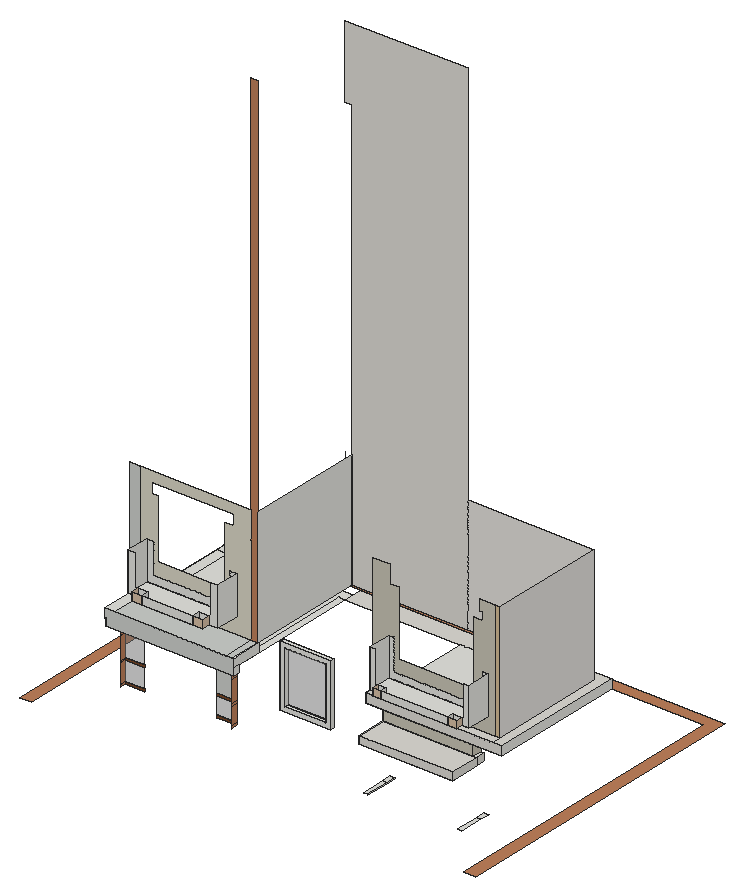
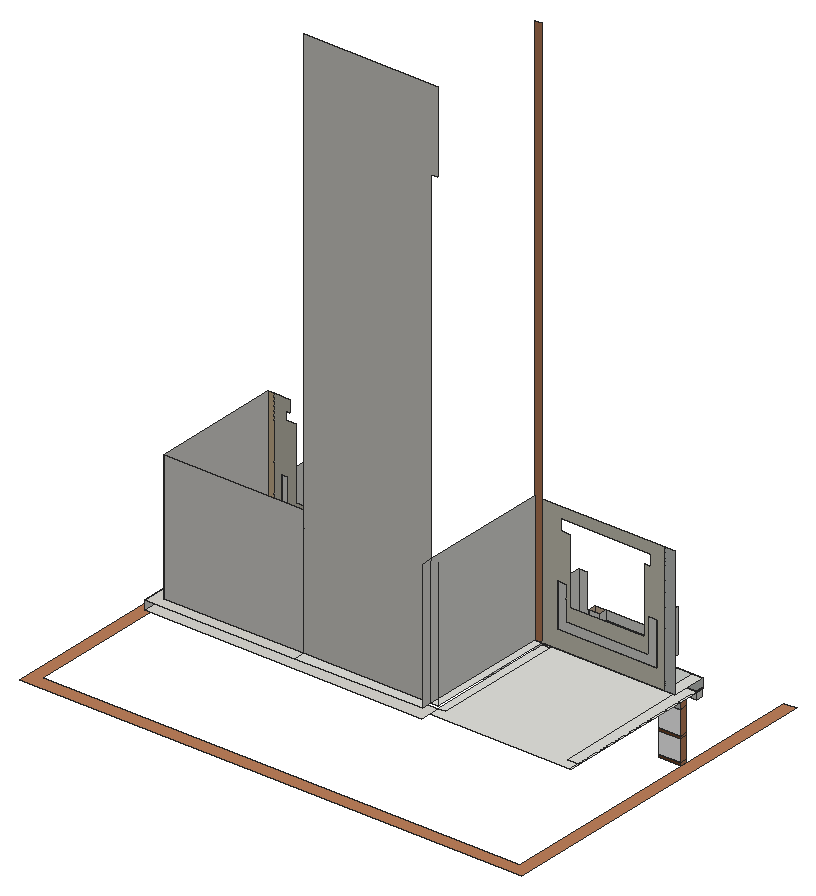
# SketchUp Ruby script. Lengths in inches.
U = 1.inch
M = Sketchup.active_model
def pt(a) = Geom::Point3d.new(a.map { |v| v * U })
def face(e, loops, mat)
  f = e.add_face(loops[0].map { |a| pt(a) })
  loops[1..].each { |l| e.add_face(l.map { |a| pt(a) }).erase! }
  f.material = f.back_material = mat if mat
  f
end
# faces: each face lists its corners as indices into pts; further lists are holes
def faces(e, pts, list, mat = nil) = list.each { |f| face(e, (f[0].is_a?(Array) ? f : [f]).map { |l| l.map { |i| pts[i] } }, mat) }
# xy, xz, yz: faces in a plane at the given z, y or x. An outline is a flat list of corners, or four numbers for a rectangle; further outlines are holes
def ring(l) = l.size == 4 ? [[l[0], l[1]], [l[2], l[1]], [l[2], l[3]], [l[0], l[3]]] : l.each_slice(2).to_a
def flat(e, list, mat, &to3) = list.each { |f| face(e, (f[0].is_a?(Array) ? f : [f]).map { |l| ring(l).map { |u, v| to3.(u, v) } }, mat) }
def xy(e, z, list, mat = nil) = flat(e, list, mat) { |x, y| [x, y, z] }
def xz(e, y, list, mat = nil) = flat(e, list, mat) { |x, z| [x, y, z] }
def yz(e, x, list, mat = nil) = flat(e, list, mat) { |y, z| [x, y, z] }
def lines(e, pts, list) = list.each { |a, b| e.add_line(pt(pts[a]), pt(pts[b])) }
# prism: a flat outline (further loops are holes) pulled along v
def prism(e, loops, v, mat = nil)
  f = face(e, loops, mat); d = Geom::Vector3d.new(v.map { |x| x * U })
  f.pushpull(f.normal.samedirection?(d) ? d.length : -d.length)
end
def box(e, o, s, mat = nil) = prism(e, [[o, [o[0] + s[0], o[1], o[2]], [o[0] + s[0], o[1] + s[1], o[2]], [o[0], o[1] + s[1], o[2]]]], [0, 0, s[2]], mat)
def at(x, y, z, deg = 0) = Geom::Transformation.translation(pt([x, y, z])) * Geom::Transformation.rotation(ORIGIN, Z_AXIS, deg.degrees)
def axes(o, x, y, z) = Geom::Transformation.new([*x, 0, *y, 0, *z, 0, *pt(o).to_a, 1])
def part(name) = M.definitions.add(name)
# library, detail: a bought-in or finely detailed component or shape, given as its bounding box
def library(name, o, s) = part(name).tap { |d| box(d.entities, o, s) }
def detail(e, o, s) = box(e.add_group.entities, o, s)
def put(e, d, t, mat = nil) = e.add_instance(d, t).tap { |i| i.material = mat if mat }
def group(e, t, mat = nil) = e.add_group.tap { |g| g.transformation = t; g.material = mat if mat }.entities
root = M.entities
M.materials.add("[Basic Tile]").color = [203, 206, 202]
M.materials.add("[Formica Beige]").color = [211, 187, 149]
M.materials.add("[Formica Graystone]").color = [198, 194, 180]
M.materials.add("[Formica Graystone]1").color = [216, 212, 196]
M.materials.add("[Formica Laminate Light]").color = [213, 189, 164]
M.materials.add("[Terrazzo Tile Accent]").color = [224, 221, 217]
M.materials.add("[Terrazzo Tile Light]").color = [219, 217, 210]
M.materials.add("[Translucent Glass Gray]").color = [128, 128, 128]
M.materials["[Translucent Glass Gray]"].alpha = 0.5
M.materials.add("[Wood Veneer 01]").color = [120, 70, 37]
M.materials.add("[Wood Veneer 02]").color = [190, 128, 91]
xy(root,63.125,[[288.3125,80.01,293.16,104.39],[384.76,80.01,389.375,104.39],[288.3125,104.39,293.16,114.1],[384.76,104.39,389.375,114.1]])
xy(root,84,[[0,0,11.79,0,11.79,307.53,455.72,307.53,455.72,0,467.51,0,467.51,319.32,0,319.32]],"[Wood Veneer 02]")
xy(root,87.4375,[[179.41,109.54,230.79,114.1]])
xy(root,91.91,[[183.89,109.54,226.3125,114.1]])
xy(root,110.81,[[375.8125,104.39,384.875,114.1]])
xy(root,110.81,[[[289.1875,73.57,384.875,104.39],[377.92,74.4375,378.51,74.59,379.03,74.88,379.47,75.3,379.77,75.82,379.9375,76.4,379.94,77.01,379.8,77.59,379.5,78.12,379.08,78.55,378.56,78.86,377.98,79.02,377.375,79.03,376.79,78.88,376.26,78.58,375.83,78.16,375.52,77.64,375.36,77.0625,375.35,76.46,375.5,75.875,375.8,75.35,376.22,74.92,376.74,74.61,377.32,74.44],[300.49,74.4375,301.07,74.59,301.6,74.88,302.03,75.3,302.34,75.82,302.5,76.4,302.51,77.01,302.36,77.59,302.0625,78.12,301.64,78.55,301.12,78.86,300.54,79.02,299.9375,79.03,299.35,78.88,298.82,78.58,298.39,78.16,298.09,77.64,297.92,77.0625,297.91,76.46,298.0625,75.875,298.36,75.35,298.78,74.92,299.3,74.61,299.88,74.44]],[289.1875,104.39,298,114.1]],"[Terrazzo Tile Light]")
xy(root,118.3125,[[381.1875,104.39,384.875,114.1]])
xy(root,118.3125,[[289.1875,73.57,384.875,104.39]],"[Terrazzo Tile Light]")
xy(root,121.75,[[22.54,82.1,22.54,88.35,32.26,88.35,32.26,94.67,146.55,94.67,146.55,88.35,153.36,88.35,153.36,82.1]])
xy(root,129,[[21.57,82.1,22.54,235.11],[22.54,88.35,32.26,225.39],[146.55,88.35,153.36,104.39],[32.26,94.67,146.55,94.67,146.55,225.39,153.36,225.39,153.36,235.11,22.54,235.11,22.54,225.39,32.26,225.39],[146.55,104.39,153.36,225.39],
  [270.97,104.39,289.1875,114.1],[289.1875,104.39,289.1875,114.1,271.94,114.1,271.94,225.39,402.13,225.39,402.13,114.1,381.1875,114.1,381.1875,104.39]])
xy(root,129,[[381.1875,104.39,381.1875,114.1,402.13,114.1,402.13,225.39,153.36,225.39,153.36,244.83,410.88,244.83,410.88,104.39]],"[Terrazzo Tile Light]")
xy(root,138,[[21.57,82.1,31.29,114.1],[152.39,82.1,153.36,114.1],[145.58,114.1,152.39,235.11],[152.39,235.11,270.97,244.83]])
xy(root,138,[[31.29,82.1,145.58,114.1],[145.58,82.1,152.39,114.1]],"[Basic Tile]")
xy(root,138,[[270.97,104.39,401.16,114.1],[401.16,104.39,410.88,104.39,410.88,244.83,270.97,244.83,270.97,235.11,401.16,235.11]],"[Terrazzo Tile Light]")
xy(root,146.65,[[183.89,109.54,226.3125,114.1]])
xy(root,151.125,[[179.41,109.54,230.79,114.1]])
xy(root,153.1875,[[303.97,83.29,303.97,89.73,287.34,89.73,287.34,114.1,388.41,114.1,388.41,89.73,372.44,89.73,372.44,83.29]])
xy(root,153.1875,[[295.13,83.29,303.97,89.73],[372.44,83.29,381.28,89.73]],"[Formica Laminate Light]")
xy(root,154.47,[[59.48,81.92,59.48,89.73,38.84,89.73,38.84,114.1,131.22,114.1,131.22,89.73,111.73,89.73,111.73,81.92]])
xy(root,154.47,[[49.36,81.92,59.48,89.73],[111.73,81.92,121.85,89.73]],"[Formica Laminate Light]")
xz(root,73.57,[[289.1875,110.81,384.875,118.3125]],"[Terrazzo Tile Light]")
xz(root,81.92,[[59.48,154.47,111.73,162.85]])
xz(root,81.92,[[49.36,154.47,59.48,162.85],[111.73,154.47,121.85,162.85]],"[Formica Laminate Light]")
xz(root,82.1,[[22.54,121.75,153.36,121.75,153.36,138,21.57,138,21.57,129,22.54,129]],"[Basic Tile]")
xz(root,83.29,[[303.97,153.1875,372.44,160.3]])
xz(root,83.29,[[295.13,153.1875,303.97,160.3],[372.44,153.1875,381.28,160.3]],"[Formica Laminate Light]")
xz(root,88.35,[[22.54,121.75,32.26,129],[146.55,121.75,153.36,129]])
xz(root,89.73,[[287.34,153.1875,295.13,153.1875,295.13,160.3,292.1875,160.3,292.1875,192.125,287.34,192.125],[295.13,153.1875,303.97,160.3],[372.44,153.1875,381.28,160.3],[381.28,153.1875,388.41,153.1875,388.41,192.125,383.79,192.125,383.79,160.3,381.28,160.3],[38.84,154.47,49.36,154.47,49.36,162.85,46.18,162.85,46.18,194.03,38.84,194.03],
  [49.36,154.47,59.48,162.85],[111.73,154.47,121.85,162.85],[121.85,154.47,131.22,154.47,131.22,194.03,123.57,194.03,123.57,162.85,121.85,162.85]])
xz(root,94.67,[[32.26,121.75,146.55,129]])
xz(root,94.67,[[126.05,90.82,146.55,113.36],[32.26,113.36,146.55,121.75]],"[Basic Tile]")
xz(root,94.67,[[32.26,68.63,52.55,88.41],[126.05,70.93,146.55,88.41],[32.26,90.82,52.55,113.36]],"[Translucent Glass Gray]")
xz(root,94.67,[[32.26,66.22,52.55,68.63],[126.05,68.52,146.55,70.93],[32.26,88.41,52.55,90.82],[126.05,88.41,146.55,90.82]],"[Wood Veneer 01]")
xz(root,104.39,[[289.1875,110.81,384.875,118.3125]])
xz(root,104.39,[[289.1875,118.3125,381.1875,129]],"[Formica Graystone]")
xz(root,104.39,[[270.97,129,410.88,138]],"[Terrazzo Tile Light]")
xz(root,109.54,[[[179.41,87.4375,230.79,151.125],[183.89,91.91,226.3125,146.65]]])
xz(root,114.1,[[[179.41,87.4375,230.79,151.125],[183.89,91.91,226.3125,146.65]],[287.34,153.1875,287.34,192.125,292.1875,192.125,292.1875,160.3,383.79,160.3,383.79,192.125,388.41,192.125,388.41,153.1875],[38.84,154.47,38.84,194.03,46.18,194.03,46.18,162.85,123.57,162.85,123.57,194.03,131.22,194.03,131.22,154.47]])
xz(root,114.1,[[21.57,138,31.29,258]],"[Basic Tile]")
xz(root,114.1,[[395.49,138,401.16,258]],"[Formica Beige]")
xz(root,114.1,[[[270.97,138,395.49,138,395.49,258,380.22,258,380.22,247.3125,383.91,247.3125,383.91,239.81,374.84,239.81,374.84,173.62,297.03,173.62,297.03,239.81,288.22,239.81,288.22,258,270.97,258],[287.34,153.1875,287.34,192.125,292.1875,192.125,292.1875,160.3,383.79,160.3,383.79,192.125,388.41,192.125,388.41,153.1875]]],"[Formica Graystone]")
xz(root,114.1,[[[31.29,138,145.58,258],[49.84,176.18,49.84,236.95,43.93,236.95,43.93,247.76,128,247.76,128,236.95,119.34,236.95,119.34,176.18],[38.84,154.47,38.84,194.03,46.18,194.03,46.18,162.85,123.57,162.85,123.57,194.03,131.22,194.03,131.22,154.47]]],"[Formica Graystone]1")
xz(root,114.1,[[183.89,91.91,226.3125,146.65]],"[Translucent Glass Gray]")
xz(root,114.1,[[145.58,138,152.39,654.5625]],"[Wood Veneer 02]")
xz(root,235.11,[[270.97,138,401.16,258]],"[Terrazzo Tile Accent]")
xz(root,235.11,[[152.39,138,152.39,579.1875,145.58,579.1875,145.58,654.5625,270.97,654.5625,270.97,138]],"[Terrazzo Tile Light]")
yz(root,22.54,[[82.1,121.75,88.35,129]])
yz(root,32.26,[[88.35,121.75,94.67,129]])
yz(root,32.26,[[88.35,66.22,94.67,68.63],[88.35,68.63,94.67,88.41],[88.35,88.41,94.67,90.82],[88.35,90.82,94.67,113.36],[88.35,113.36,94.67,121.75]],"[Wood Veneer 02]")
yz(root,38.84,[[89.73,154.47,114.1,194.03]])
yz(root,49.36,[[81.92,154.47,89.73,162.85]],"[Formica Laminate Light]")
yz(root,59.48,[[81.92,154.47,89.73,162.85]])
yz(root,111.73,[[81.92,154.47,89.73,162.85]])
yz(root,121.85,[[81.92,154.47,89.73,162.85]],"[Formica Laminate Light]")
yz(root,131.22,[[89.73,154.47,114.1,194.03]])
yz(root,146.55,[[88.35,121.75,94.67,129]])
yz(root,146.55,[[88.35,68.52,94.67,70.93],[88.35,70.93,94.67,88.41],[88.35,88.41,94.67,90.82],[88.35,90.82,94.67,113.36],[88.35,113.36,94.67,121.75]],"[Wood Veneer 02]")
yz(root,152.39,[[114.1,138,235.11,258]])
yz(root,152.39,[[235.11,138,244.83,258]],"[Terrazzo Tile Accent]")
yz(root,153.36,[[82.1,121.75,88.35,129],[82.1,129,114.1,138]])
yz(root,179.41,[[109.54,87.4375,114.1,151.125]])
yz(root,183.89,[[109.54,91.91,114.1,146.65]])
yz(root,226.3125,[[109.54,91.91,114.1,146.65]])
yz(root,230.79,[[109.54,87.4375,114.1,151.125]])
yz(root,270.97,[[104.39,129,114.1,138]])
yz(root,287.34,[[89.73,153.1875,114.1,192.125]])
yz(root,289.1875,[[104.39,110.81,114.1,118.3125],[104.39,118.3125,114.1,129]],"[Formica Graystone]")
yz(root,289.1875,[[73.57,110.81,104.39,118.3125]],"[Terrazzo Tile Light]")
yz(root,293.16,[[80.01,62.16,104.39,63.125],[104.39,62.16,114.1,63.125]])
yz(root,295.13,[[83.29,153.1875,89.73,160.3]],"[Formica Laminate Light]")
yz(root,303.97,[[83.29,153.1875,89.73,160.3]])
yz(root,372.44,[[83.29,153.1875,89.73,160.3]])
yz(root,381.1875,[[104.39,118.3125,114.1,129]],"[Formica Graystone]")
yz(root,381.28,[[83.29,153.1875,89.73,160.3]],"[Formica Laminate Light]")
yz(root,384.875,[[73.57,110.81,104.39,118.3125],[104.39,110.81,114.1,118.3125]],"[Terrazzo Tile Light]")
yz(root,388.41,[[89.73,153.1875,114.1,192.125]])
yz(root,401.16,[[114.1,138,235.11,258]],"[Terrazzo Tile Accent]")
yz(root,410.88,[[104.39,129,244.83,138]])
p = [[145.58,235.11,138],[145.58,235.11,258]]
lines(root,p,[[0,1]])
